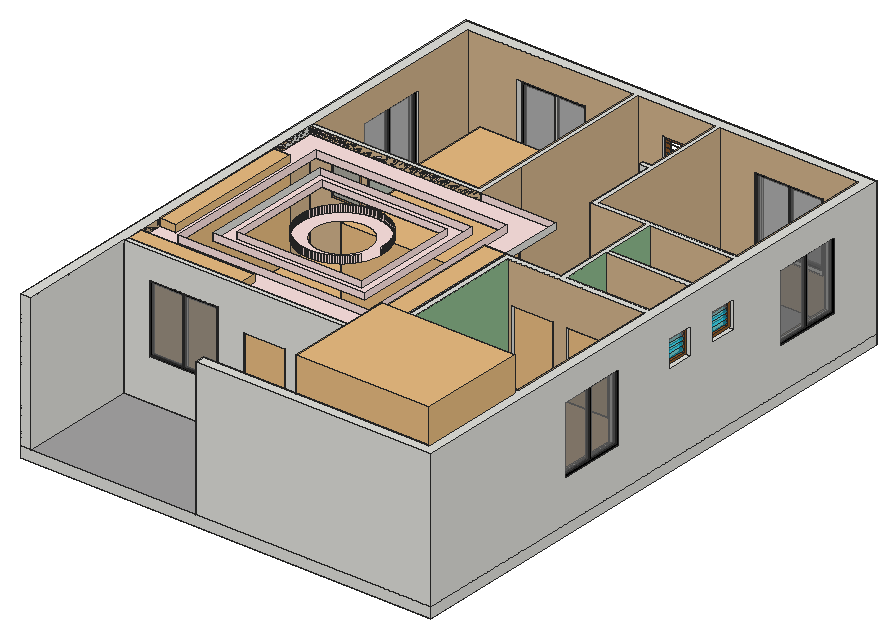
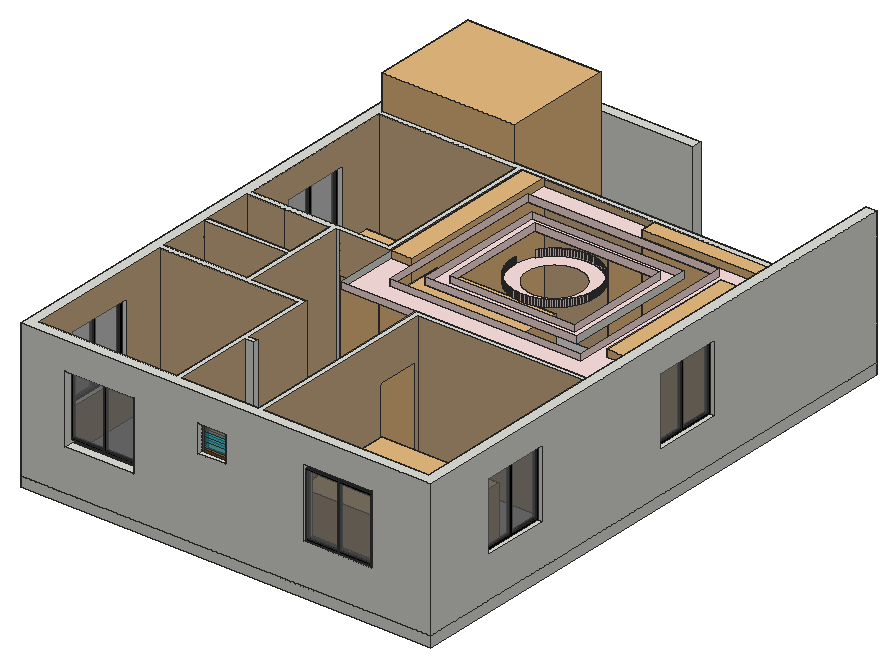
# SketchUp Ruby script. Lengths in inches.
U = 1.inch
M = Sketchup.active_model
def pt(a) = Geom::Point3d.new(a.map { |v| v * U })
def face(e, loops, mat)
  f = e.add_face(loops[0].map { |a| pt(a) })
  loops[1..].each { |l| e.add_face(l.map { |a| pt(a) }).erase! }
  f.material = f.back_material = mat if mat
  f
end
# faces: each face lists its corners as indices into pts; further lists are holes
def faces(e, pts, list, mat = nil) = list.each { |f| face(e, (f[0].is_a?(Array) ? f : [f]).map { |l| l.map { |i| pts[i] } }, mat) }
# xy, xz, yz: faces in a plane at the given z, y or x. An outline is a flat list of corners, or four numbers for a rectangle; further outlines are holes
def ring(l) = l.size == 4 ? [[l[0], l[1]], [l[2], l[1]], [l[2], l[3]], [l[0], l[3]]] : l.each_slice(2).to_a
def flat(e, list, mat, &to3) = list.each { |f| face(e, (f[0].is_a?(Array) ? f : [f]).map { |l| ring(l).map { |u, v| to3.(u, v) } }, mat) }
def xy(e, z, list, mat = nil) = flat(e, list, mat) { |x, y| [x, y, z] }
def xz(e, y, list, mat = nil) = flat(e, list, mat) { |x, z| [x, y, z] }
def yz(e, x, list, mat = nil) = flat(e, list, mat) { |y, z| [x, y, z] }
def lines(e, pts, list) = list.each { |a, b| e.add_line(pt(pts[a]), pt(pts[b])) }
# prism: a flat outline (further loops are holes) pulled along v
def prism(e, loops, v, mat = nil)
  f = face(e, loops, mat); d = Geom::Vector3d.new(v.map { |x| x * U })
  f.pushpull(f.normal.samedirection?(d) ? d.length : -d.length)
end
def box(e, o, s, mat = nil) = prism(e, [[o, [o[0] + s[0], o[1], o[2]], [o[0] + s[0], o[1] + s[1], o[2]], [o[0], o[1] + s[1], o[2]]]], [0, 0, s[2]], mat)
def at(x, y, z, deg = 0) = Geom::Transformation.translation(pt([x, y, z])) * Geom::Transformation.rotation(ORIGIN, Z_AXIS, deg.degrees)
def axes(o, x, y, z) = Geom::Transformation.new([*x, 0, *y, 0, *z, 0, *pt(o).to_a, 1])
def part(name) = M.definitions.add(name)
# library, detail: a bought-in or finely detailed component or shape, given as its bounding box
def library(name, o, s) = part(name).tap { |d| box(d.entities, o, s) }
def detail(e, o, s) = box(e.add_group.entities, o, s)
def put(e, d, t, mat = nil) = e.add_instance(d, t).tap { |i| i.material = mat if mat }
def group(e, t, mat = nil) = e.add_group.tap { |g| g.transformation = t; g.material = mat if mat }.entities
root = M.entities
M.materials.add("F10").color = [176, 183, 172]
M.materials.add("F11").color = [173, 179, 169]
M.materials.add("F20").color = [169, 167, 158]
M.materials.add("Querkus Oak Naturel Adagio _ Architonic1").color = [173, 130, 81]
M.materials.add("[0007_MistyRose]").color = [255, 228, 225]
M.materials.add("[0010_Snow]").color = [255, 250, 250]
M.materials.add("[0035_Tan]").color = [210, 180, 140]
M.materials.add("[0057_DarkKhaki]").color = [189, 183, 107]
M.materials.add("[0072_DarkSeaGreen]").color = [143, 188, 143]
M.materials.add("[Carrera Marble]").color = [207, 207, 207]
M.materials.add("[Color_008]").color = [30, 30, 30]
M.materials.add("[Color_009]").color = [0, 0, 0]
M.materials.add("[Stone Vein Gray]").color = [166, 165, 165]
M.materials.add("[Translucent Glass Gray]").color = [128, 128, 128]
M.materials["[Translucent Glass Gray]"].alpha = 0.5
M.materials.add("[Translucent Glass Tinted]1").color = [7, 201, 240]
M.materials["[Translucent Glass Tinted]1"].alpha = 0.48
M.materials.add("[Translucent_Glass_Gray]").color = [128, 128, 128]
M.materials["[Translucent_Glass_Gray]"].alpha = 0.5
M.materials.add("[Wood Cherry Original]").color = [152, 86, 42]
M.materials.add("[Wood Floor Parquet]").color = [145, 89, 39]
c1 = library("Group\#5",[0,0,0],[116.44,93.99,154.6875])
c2 = library("Senza",[-40.91,-66.2,-0.5],[133.3,90.15,38.26])
c3 = library("Modern+dining",[-0.9,-1.38,-0.1],[126.72,78.33,130.86])
c4 = library("main+door",[0,-0.79,0],[47.24,7.88,82.68])
c5 = library("Bed",[-100.55,9.74,0],[90.43,103.1,58.68])
c6 = library("CS300DRT",[0,0,0],[27.18,17.85,30.31])
c7 = part("ventilator")
g1 = group(c7.entities,at(0,0,0))
xy(g1,0,[[0,0,24,1],[0,1,24,6.83]],"[Wood Floor Parquet]")
xy(g1,1.75,[[2,0,22,6.83]],"[Wood Floor Parquet]")
xy(g1,21.87,[[2,0,22,6.83]],"[Wood Cherry Original]")
xy(g1,23.62,[[0,0,24,1],[0,1,24,6.83]],"[Wood Floor Parquet]")
xz(g1,0,[[[0,0,24,23.62],[2,1.75,22,21.87]]],"[Wood Floor Parquet]")
xz(g1,6.83,[[[0,0,24,23.62],[2,1.75,22,21.87]]],"[Wood Cherry Original]")
yz(g1,0,[[0,0,1,23.62],[1,0,6.83,23.62]],"[Wood Floor Parquet]")
yz(g1,2,[[0,1.75,6.83,1.75,6.83,7.66,0,3.5],[0,3.5,6.83,7.66,6.83,11.8125,0,7.66],[0,7.66,6.83,11.8125,6.83,15.97,0,11.8125],[0,11.8125,6.83,15.97,6.83,20.12,0,15.97],[0,15.97,6.83,20.12,6.83,21.87,0,21.87]],"[Wood Floor Parquet]")
yz(g1,22,[[0,1.75,0,3.5,6.83,7.66,6.83,1.75],[0,3.5,0,7.66,6.83,11.8125,6.83,7.66],[0,7.66,0,11.8125,6.83,15.97,6.83,11.8125],[0,11.8125,0,15.97,6.83,20.12,6.83,15.97],[0,15.97,0,21.87,6.83,21.87,6.83,20.12]],"[Wood Floor Parquet]")
yz(g1,24,[[0,0,1,23.62],[1,0,6.83,23.62]],"[Wood Floor Parquet]")
p = [[2,0,3.5],[2,6.83,7.66],[22,6.83,7.66],[22,0,3.5],[2,6.83,11.8125],[2,0,7.66],
  [22,0,7.66],[22,6.83,11.8125],[2,0,11.8125],[2,6.83,15.97],[22,6.83,15.97],[22,0,11.8125],
  [2,6.83,20.12],[2,0,15.97],[22,0,15.97],[22,6.83,20.12]]
faces(g1,p,[[0,1,2,3],[4,5,6,7],[8,9,10,11]],"[Translucent Glass Tinted]1")
faces(g1,p,[[12,13,14,15]],"[Translucent Glass Gray]")
c8 = part("Group\#2")
xy(c8.entities,0,[[0,0,82.68,1.18]],"[Color_009]")
xy(c8.entities,1.97,[[1.97,0.98,40.35,1.18],[42.32,0.98,80.71,1.18]])
xy(c8.entities,1.97,[[1.97,0,40.35,0.3],[42.32,0,80.71,0.3]],"[Color_009]")
xy(c8.entities,80.71,[[1.97,0,40.35,0.3],[42.32,0,80.71,0.3],[1.97,0.3,40.35,0.98],[42.32,0.3,80.71,0.98],[1.97,0.98,40.35,1.18],
  [42.32,0.98,80.71,1.18]])
xy(c8.entities,82.68,[[0,0,82.68,1.18]],"[Color_008]")
xz(c8.entities,0,[[[0,0,82.68,82.68],[1.97,1.97,40.35,80.71],[42.32,1.97,80.71,80.71]]],"[Color_009]")
xz(c8.entities,0.3,[[1.97,1.97,40.35,80.71],[42.32,1.97,80.71,80.71]],"[Translucent_Glass_Gray]")
xz(c8.entities,0.98,[[1.97,1.97,40.35,80.71],[42.32,1.97,80.71,80.71]],"[Translucent_Glass_Gray]")
xz(c8.entities,1.18,[[[0,0,82.68,82.68],[1.97,1.97,80.71,80.71]],[40.35,1.97,42.32,80.71]],"[Color_009]")
yz(c8.entities,0,[[0,0,1.18,82.68]],"[Color_009]")
yz(c8.entities,1.97,[[0.98,1.97,1.18,80.71]])
yz(c8.entities,1.97,[[0,1.97,0.3,80.71]],"[Color_009]")
yz(c8.entities,40.35,[[0,1.97,0.3,80.71],[0.98,1.97,1.18,80.71]],"[Color_009]")
yz(c8.entities,42.32,[[0,1.97,0.3,80.71],[0.98,1.97,1.18,80.71]])
yz(c8.entities,80.71,[[0,1.97,0.3,80.71],[0.98,1.97,1.18,80.71]],"[Color_009]")
yz(c8.entities,82.68,[[0,0,1.18,82.68]],"[Color_009]")
c9 = library("Group\#28",[0,0,0],[19.5,144,120])
c10 = library("Platform bed",[0,0,0],[83.59,112.46,35.43])
c11 = library("Curtains and rod",[2.63,-1.46,0.02],[153.32,14.02,114.15])
c12 = library("SKT_Nearly Natural 5' Kentia Palm Silk Tree",[-23.18,-17.61,0],[47.48,43.95,59.125])
c13 = library("Round wall hanging",[0,0,0],[26.88,1.18,49.49])
c14 = part("Group\#37")
prism(c14.entities,[[[0,0.6,0],[0,0.6,24.5],[19,0.6,24.5],[19,0.6,0]],[[0.5,0.6,0.5],[18.5,0.6,0.5],[18.5,0.6,24],[0.5,0.6,24]]],[0,-0.6,0])
c15 = part("F9")
g2 = group(c15.entities,at(48,0,0))
xy(g2,0.5,[[0.5,0.3,18.5,0.6]])
xy(g2,24,[[0.5,0.3,18.5,0.6]])
xz(g2,0.3,[[0.5,0.5,18.5,24]],"F11")
xz(g2,0.6,[[0.5,0.5,18.5,24]],"[0010_Snow]")
yz(g2,0.5,[[0.3,0.5,0.6,24]])
yz(g2,18.5,[[0.3,0.5,0.6,24]])
put(g2,c14,axes([19,0,0],[-1,0,0],[0,1,0],[0,0,1]),"Querkus Oak Naturel Adagio _ Architonic1")
g3 = group(c15.entities,at(24,0,0))
xy(g3,0.5,[[0.5,0.3,18.5,0.6]])
xy(g3,24,[[0.5,0.3,18.5,0.6]])
xz(g3,0.3,[[0.5,0.5,18.5,24]],"F10")
xz(g3,0.6,[[0.5,0.5,18.5,24]],"[0010_Snow]")
yz(g3,0.5,[[0.3,0.5,0.6,24]])
yz(g3,18.5,[[0.3,0.5,0.6,24]])
put(g3,c14,axes([19,0,0],[-1,0,0],[0,1,0],[0,0,1]),"Querkus Oak Naturel Adagio _ Architonic1")
g4 = group(c15.entities,at(0,0,0))
xy(g4,0.5,[[0.5,0.3,18.5,0.6]])
xy(g4,24,[[0.5,0.3,18.5,0.6]])
xz(g4,0.3,[[0.5,0.5,18.5,24]],"F20")
xz(g4,0.6,[[0.5,0.5,18.5,24]],"[0010_Snow]")
yz(g4,0.5,[[0.3,0.5,0.6,24]])
yz(g4,18.5,[[0.3,0.5,0.6,24]])
put(g4,c14,axes([19,0,0],[-1,0,0],[0,1,0],[0,0,1]),"Querkus Oak Naturel Adagio _ Architonic1")
xy(root,114,[[[9,107.25,224.75,306.75],[33,131.25,200.75,282.75]],[[50.24,148.49,183.51,265.51],[62.05,160.3,171.7,253.7]],[[116.7,171,115.57,171.02,114.44,171.08,113.3125,171.18,112.19,171.31,111.07,171.47,109.96,171.67,108.85,171.91,107.75,172.17,106.66,172.48,105.58,172.82,104.52,173.1875,103.46,173.59,102.42,174.03,101.39,174.5,100.375,175,99.38,175.54,98.4,176.1,97.4375,176.7,96.5,177.32,95.57,177.98,94.67,178.66,93.79,179.37,92.9375,180.11,92.1,180.875,91.3,181.67,90.51,182.48,89.76,183.32,89.03,184.1875,88.32,185.07,87.65,185.98,87,186.91,86.39,187.86,85.8,188.82,85.24,189.81,84.72,190.8125,84.23,191.83,83.77,192.86,83.34,193.91,82.94,194.97,82.58,196.04,82.26,197.125,81.96,198.22,81.7,199.32,81.48,200.43,81.29,201.54,81.14,202.66,81.02,203.79,80.9375,204.91,80.89,206.04,80.875,207.17,80.9,208.3,80.96,209.43,81.05,210.5625,81.18,211.68,81.35,212.8,81.55,213.92,81.78,215.02,82.05,216.12,82.35,217.21,82.69,218.29,83.0625,219.36,83.47,220.41,83.91,221.46,84.375,222.49,84.88,223.5,85.41,224.5,85.98,225.48,86.57,226.4375,87.2,227.38,87.85,228.3,88.54,229.2,89.25,230.08,89.99,230.9375,90.75,231.77,91.54,232.58,92.36,233.36,93.2,234.12,94.0625,234.85,94.95,235.55,95.86,236.23,96.78,236.87,97.73,237.49,98.7,238.08,99.68,238.63,100.6875,239.15,101.7,239.65,102.74,240.11,103.78,240.54,104.84,240.93,105.92,241.29,107,241.62,108.09,241.91,109.19,242.17,110.3,242.39,111.42,242.58,112.54,242.74,113.66,242.86,114.79,242.9375,115.92,242.99,117.05,243,118.18,242.98,119.31,242.92,120.4375,242.82,121.56,242.69,122.68,242.53,123.79,242.33,124.9,242.09,126,241.83,127.09,241.52,128.17,241.18,129.23,240.8125,130.29,240.41,131.33,239.97,132.36,239.5,133.375,239,134.37,238.46,135.35,237.9,136.3125,237.3,137.25,236.68,138.18,236.02,139.08,235.34,139.96,234.63,140.8125,233.89,141.65,233.125,142.45,232.33,143.24,231.52,143.99,230.68,144.72,229.8125,145.43,228.93,146.1,228.02,146.75,227.09,147.36,226.14,147.95,225.18,148.51,224.19,149.03,223.1875,149.52,222.17,149.98,221.14,150.41,220.09,150.81,219.03,151.17,217.96,151.49,216.875,151.79,215.78,152.05,214.68,152.27,213.57,152.46,212.46,152.61,211.34,152.73,210.21,152.8125,209.09,152.86,207.96,152.875,206.83,152.85,205.7,152.79,204.57,152.7,203.4375,152.57,202.32,152.4,201.2,152.2,200.08,151.97,198.98,151.7,197.88,151.4,196.79,151.06,195.71,150.6875,194.64,150.28,193.59,149.84,192.54,149.375,191.51,148.87,190.5,148.34,189.5,147.77,188.52,147.18,187.5625,146.55,186.62,145.9,185.7,145.21,184.8,144.5,183.92,143.76,183.0625,143,182.23,142.21,181.42,141.39,180.64,140.55,179.88,139.6875,179.15,138.8,178.45,137.89,177.77,136.97,177.13,136.02,176.51,135.05,175.92,134.07,175.37,133.0625,174.85,132.05,174.35,131.01,173.89,129.97,173.46,128.91,173.07,127.83,172.71,126.75,172.38,125.66,172.09,124.56,171.83,123.45,171.61,122.33,171.42,121.21,171.26,120.09,171.14,118.96,171.0625,117.83,171.01],[116.59,183,117.34,183,118.1,183.03,118.85,183.08,119.6,183.15,120.35,183.25,121.09,183.37,121.83,183.52,122.56,183.68,123.29,183.875,124.02,184.09,124.73,184.32,125.44,184.58,126.14,184.86,126.83,185.16,127.51,185.49,128.18,185.83,128.84,186.2,129.49,186.58,130.125,186.99,130.75,187.42,131.36,187.86,131.95,188.33,132.53,188.81,133.09,189.31,133.64,189.83,134.17,190.36,134.6875,190.91,135.18,191.48,135.66,192.0625,136.12,192.66,136.5625,193.27,136.98,193.9,137.39,194.54,137.77,195.1875,138.13,195.85,138.47,196.52,138.79,197.21,139.08,197.9,139.36,198.6,139.61,199.3125,139.84,200.03,140.05,200.75,140.23,201.48,140.39,202.22,140.53,202.96,140.65,203.71,140.74,204.46,140.81,205.21,140.85,205.96,140.875,206.71,140.87,207.47,140.84,208.22,140.79,208.97,140.72,209.72,140.62,210.47,140.5,211.21,140.36,211.95,140.19,212.69,140,213.42,139.79,214.14,139.55,214.86,139.29,215.57,139.01,216.27,138.71,216.96,138.39,217.64,138.04,218.31,137.68,218.97,137.29,219.62,136.89,220.25,136.46,220.875,136.01,221.48,135.55,222.08,135.07,222.65,134.57,223.22,134.05,223.77,133.51,224.3,132.96,224.8125,132.39,225.31,131.8125,225.79,131.21,226.25,130.6,226.6875,129.98,227.11,129.34,227.51,128.6875,227.89,128.03,228.25,127.35,228.59,126.67,228.91,125.98,229.21,125.27,229.48,124.5625,229.73,123.85,229.97,123.12,230.17,122.39,230.36,121.65,230.52,120.91,230.66,120.17,230.77,119.42,230.86,118.67,230.93,117.92,230.98,117.16,231,116.41,231,115.65,230.97,114.9,230.92,114.15,230.85,113.4,230.75,112.66,230.63,111.92,230.48,111.19,230.32,110.46,230.125,109.73,229.91,109.02,229.68,108.31,229.42,107.61,229.14,106.92,228.84,106.24,228.51,105.57,228.17,104.91,227.8,104.26,227.42,103.625,227.01,103,226.58,102.39,226.14,101.8,225.67,101.22,225.19,100.66,224.69,100.11,224.17,99.58,223.64,99.0625,223.09,98.57,222.52,98.09,221.9375,97.63,221.34,97.1875,220.73,96.77,220.1,96.36,219.46,95.98,218.8125,95.62,218.15,95.28,217.48,94.96,216.79,94.67,216.1,94.39,215.4,94.14,214.6875,93.91,213.97,93.7,213.25,93.52,212.52,93.36,211.78,93.22,211.04,93.1,210.29,93.01,209.54,92.94,208.79,92.9,208.04,92.875,207.29,92.88,206.53,92.91,205.78,92.96,205.03,93.03,204.28,93.13,203.53,93.25,202.79,93.39,202.05,93.56,201.31,93.75,200.58,93.96,199.86,94.2,199.14,94.46,198.43,94.74,197.73,95.04,197.04,95.36,196.36,95.71,195.69,96.07,195.03,96.46,194.38,96.86,193.75,97.29,193.125,97.74,192.52,98.2,191.92,98.68,191.35,99.18,190.78,99.7,190.23,100.24,189.7,100.79,189.1875,101.36,188.69,101.9375,188.21,102.54,187.75,103.15,187.3125,103.77,186.89,104.41,186.49,105.0625,186.11,105.72,185.75,106.4,185.41,107.08,185.09,107.77,184.79,108.48,184.52,109.1875,184.27,109.9,184.03,110.63,183.83,111.36,183.64,112.1,183.48,112.84,183.34,113.58,183.23,114.33,183.14,115.08,183.07,115.83,183.02]]],"[0007_MistyRose]")
xz(root,107.25,[[9,114,224.75,120]])
xz(root,131.25,[[33,114,200.75,120]],"[0007_MistyRose]")
xz(root,148.49,[[50.24,114,183.51,120]],"[0007_MistyRose]")
xz(root,160.3,[[62.05,114,171.7,120]],"[0007_MistyRose]")
xz(root,253.7,[[62.05,114,171.7,120]],"[0007_MistyRose]")
xz(root,265.51,[[50.24,114,183.51,120]],"[0007_MistyRose]")
xz(root,282.75,[[33,114,200.75,120]],"[0007_MistyRose]")
xz(root,306.75,[[9,114,224.75,120]],"[0007_MistyRose]")
yz(root,9,[[107.25,114,306.75,120]])
yz(root,33,[[131.25,114,282.75,120]],"[0007_MistyRose]")
yz(root,50.24,[[148.49,114,265.51,120]])
yz(root,62.05,[[160.3,114,253.7,120]],"[0007_MistyRose]")
yz(root,171.7,[[160.3,114,253.7,120]],"[0007_MistyRose]")
yz(root,183.51,[[148.49,114,265.51,120]],"[0007_MistyRose]")
yz(root,200.75,[[131.25,114,282.75,120]],"[0007_MistyRose]")
yz(root,224.75,[[107.25,114,306.75,120]])
p = [[115.57,171.02,120],[114.44,171.08,120],[114.44,171.08,114],[115.57,171.02,114],[116.7,171,120],[116.7,171,114],
  [117.83,171.01,120],[117.83,171.01,114],[118.96,171.0625,120],[118.96,171.0625,114],[113.3125,171.18,120],[113.3125,171.18,114],
  [120.09,171.14,120],[120.09,171.14,114],[121.21,171.26,120],[121.21,171.26,114],[112.19,171.31,120],[112.19,171.31,114],
  [111.07,171.47,120],[111.07,171.47,114],[122.33,171.42,120],[122.33,171.42,114],[123.45,171.61,120],[123.45,171.61,114],
  [109.96,171.67,120],[109.96,171.67,114],[124.56,171.83,120],[124.56,171.83,114],[108.85,171.91,120],[108.85,171.91,114],
  [125.66,172.09,120],[125.66,172.09,114],[107.75,172.17,120],[107.75,172.17,114],[126.75,172.38,120],[126.75,172.38,114],
  [106.66,172.48,120],[106.66,172.48,114],[127.83,172.71,120],[127.83,172.71,114],[105.58,172.82,120],[105.58,172.82,114],
  [128.91,173.07,120],[128.91,173.07,114],[104.52,173.1875,120],[104.52,173.1875,114],[129.97,173.46,120],[129.97,173.46,114],
  [103.46,173.59,120],[103.46,173.59,114],[131.01,173.89,120],[131.01,173.89,114],[102.42,174.03,120],[102.42,174.03,114],
  [132.05,174.35,120],[132.05,174.35,114],[101.39,174.5,120],[101.39,174.5,114],[133.0625,174.85,120],[133.0625,174.85,114],
  [100.375,175,120],[100.375,175,114],[134.07,175.37,120],[134.07,175.37,114],[99.38,175.54,120],[99.38,175.54,114],
  [135.05,175.92,120],[135.05,175.92,114],[98.4,176.1,120],[98.4,176.1,114],[136.02,176.51,120],[136.02,176.51,114],
  [97.4375,176.7,120],[97.4375,176.7,114],[136.97,177.13,120],[136.97,177.13,114],[96.5,177.32,120],[96.5,177.32,114],
  [137.89,177.77,120],[137.89,177.77,114],[95.57,177.98,120],[95.57,177.98,114],[138.8,178.45,120],[138.8,178.45,114],
  [94.67,178.66,120],[94.67,178.66,114],[139.6875,179.15,120],[139.6875,179.15,114],[93.79,179.37,120],[93.79,179.37,114],
  [140.55,179.88,120],[140.55,179.88,114],[92.9375,180.11,120],[92.9375,180.11,114],[141.39,180.64,120],[141.39,180.64,114],
  [92.1,180.875,120],[92.1,180.875,114],[142.21,181.42,120],[142.21,181.42,114],[91.3,181.67,120],[91.3,181.67,114],
  [143,182.23,120],[143,182.23,114],[90.51,182.48,120],[90.51,182.48,114],[143.76,183.0625,120],[143.76,183.0625,114],
  [89.76,183.32,120],[89.76,183.32,114],[144.5,183.92,120],[144.5,183.92,114],[89.03,184.1875,120],[89.03,184.1875,114],
  [145.21,184.8,120],[145.21,184.8,114],[88.32,185.07,120],[88.32,185.07,114],[145.9,185.7,120],[145.9,185.7,114],
  [87.65,185.98,120],[87.65,185.98,114],[146.55,186.62,120],[146.55,186.62,114],[87,186.91,120],[87,186.91,114],
  [147.18,187.5625,120],[147.18,187.5625,114],[86.39,187.86,120],[86.39,187.86,114],[147.77,188.52,120],[147.77,188.52,114],
  [85.8,188.82,120],[85.8,188.82,114],[85.24,189.81,120],[85.24,189.81,114],[84.72,190.8125,120],[84.72,190.8125,114],
  [84.23,191.83,120],[84.23,191.83,114],[83.77,192.86,120],[83.77,192.86,114],[83.34,193.91,120],[83.34,193.91,114],
  [82.94,194.97,120],[82.94,194.97,114],[82.58,196.04,120],[82.58,196.04,114],[82.26,197.125,120],[82.26,197.125,114],
  [81.96,198.22,120],[81.96,198.22,114],[81.7,199.32,120],[81.7,199.32,114],[81.48,200.43,120],[81.48,200.43,114],
  [81.29,201.54,120],[81.29,201.54,114],[81.14,202.66,120],[81.14,202.66,114],[81.02,203.79,120],[81.02,203.79,114],
  [80.9375,204.91,120],[80.9375,204.91,114],[152.85,205.7,120],[152.79,204.57,120],[152.79,204.57,114],[152.85,205.7,114],
  [80.89,206.04,120],[80.89,206.04,114],[152.875,206.83,120],[152.875,206.83,114],[80.875,207.17,120],[80.875,207.17,114],
  [152.86,207.96,120],[152.86,207.96,114],[80.9,208.3,120],[80.9,208.3,114],[152.8125,209.09,120],[152.8125,209.09,114],
  [80.96,209.43,120],[80.96,209.43,114],[152.73,210.21,120],[152.73,210.21,114],[81.05,210.5625,120],[81.05,210.5625,114],
  [152.61,211.34,120],[152.61,211.34,114],[81.18,211.68,120],[81.18,211.68,114],[152.46,212.46,120],[152.46,212.46,114],
  [81.35,212.8,120],[81.35,212.8,114],[152.27,213.57,120],[152.27,213.57,114],[81.55,213.92,120],[81.55,213.92,114],
  [152.05,214.68,120],[152.05,214.68,114],[81.78,215.02,120],[81.78,215.02,114],[151.79,215.78,120],[151.79,215.78,114],
  [82.05,216.12,120],[82.05,216.12,114],[151.49,216.875,120],[151.49,216.875,114],[82.35,217.21,120],[82.35,217.21,114],
  [151.17,217.96,120],[151.17,217.96,114],[82.69,218.29,120],[82.69,218.29,114],[150.81,219.03,120],[150.81,219.03,114],
  [83.0625,219.36,120],[83.0625,219.36,114],[150.41,220.09,120],[150.41,220.09,114],[83.47,220.41,120],[83.47,220.41,114],
  [149.98,221.14,120],[149.98,221.14,114],[83.91,221.46,120],[83.91,221.46,114],[149.52,222.17,120],[149.52,222.17,114],
  [84.375,222.49,120],[84.375,222.49,114],[149.03,223.1875,120],[149.03,223.1875,114],[84.88,223.5,120],[84.88,223.5,114],
  [148.51,224.19,120],[148.51,224.19,114],[85.41,224.5,120],[85.41,224.5,114],[147.95,225.18,120],[147.95,225.18,114],
  [85.98,225.48,120],[85.98,225.48,114],[147.36,226.14,120],[147.36,226.14,114],[86.57,226.4375,120],[86.57,226.4375,114],
  [146.75,227.09,120],[146.75,227.09,114],[87.2,227.38,120],[87.2,227.38,114],[146.1,228.02,120],[146.1,228.02,114],
  [87.85,228.3,120],[87.85,228.3,114],[145.43,228.93,120],[145.43,228.93,114],[88.54,229.2,120],[88.54,229.2,114],
  [144.72,229.8125,120],[144.72,229.8125,114],[89.25,230.08,120],[89.25,230.08,114],[143.99,230.68,120],[143.99,230.68,114],
  [89.99,230.9375,120],[89.99,230.9375,114],[143.24,231.52,120],[143.24,231.52,114],[90.75,231.77,120],[90.75,231.77,114],
  [142.45,232.33,120],[142.45,232.33,114],[91.54,232.58,120],[91.54,232.58,114],[141.65,233.125,120],[141.65,233.125,114],
  [92.36,233.36,120],[92.36,233.36,114],[140.8125,233.89,120],[140.8125,233.89,114],[93.2,234.12,120],[93.2,234.12,114],
  [139.96,234.63,120],[139.96,234.63,114],[94.0625,234.85,120],[94.0625,234.85,114],[139.08,235.34,120],[139.08,235.34,114],
  [94.95,235.55,120],[94.95,235.55,114],[138.18,236.02,120],[138.18,236.02,114],[95.86,236.23,120],[95.86,236.23,114],
  [137.25,236.68,120],[137.25,236.68,114],[96.78,236.87,120],[96.78,236.87,114],[136.3125,237.3,120],[136.3125,237.3,114],
  [97.73,237.49,120],[97.73,237.49,114],[135.35,237.9,120],[135.35,237.9,114],[98.7,238.08,120],[98.7,238.08,114],
  [134.37,238.46,120],[134.37,238.46,114],[99.68,238.63,120],[99.68,238.63,114],[133.375,239,120],[133.375,239,114],
  [100.6875,239.15,120],[100.6875,239.15,114],[132.36,239.5,120],[132.36,239.5,114],[101.7,239.65,120],[101.7,239.65,114],
  [131.33,239.97,120],[131.33,239.97,114],[102.74,240.11,120],[102.74,240.11,114],[130.29,240.41,120],[130.29,240.41,114],
  [103.78,240.54,120],[103.78,240.54,114],[129.23,240.8125,120],[129.23,240.8125,114],[104.84,240.93,120],[104.84,240.93,114],
  [128.17,241.18,120],[128.17,241.18,114],[105.92,241.29,120],[105.92,241.29,114],[127.09,241.52,120],[127.09,241.52,114],
  [107,241.62,120],[107,241.62,114],[126,241.83,120],[126,241.83,114],[108.09,241.91,120],[108.09,241.91,114],
  [124.9,242.09,120],[124.9,242.09,114],[109.19,242.17,120],[109.19,242.17,114],[123.79,242.33,120],[123.79,242.33,114],
  [110.3,242.39,120],[110.3,242.39,114],[122.68,242.53,120],[122.68,242.53,114],[111.42,242.58,120],[111.42,242.58,114],
  [121.56,242.69,120],[121.56,242.69,114],[112.54,242.74,120],[112.54,242.74,114],[113.66,242.86,120],[113.66,242.86,114],
  [120.4375,242.82,120],[120.4375,242.82,114],[119.31,242.92,120],[119.31,242.92,114],[114.79,242.9375,120],[114.79,242.9375,114],
  [115.92,242.99,120],[115.92,242.99,114],[118.18,242.98,120],[118.18,242.98,114],[117.05,243,120],[117.05,243,114],
  [158.25,410.25,0],[158.27,410.25,0],[158.25,405.75,0],[158.27,405.75,0]]
faces(root,p,[[0,1,2,3],[4,0,3,5],[6,4,5,7],[8,6,7,9],[1,10,11,2],[12,8,9,13],[14,12,13,15],[10,16,17,11],
  [16,18,19,17],[20,14,15,21],[22,20,21,23],[18,24,25,19],[26,22,23,27],[24,28,29,25],[30,26,27,31],[28,32,33,29],
  [34,30,31,35],[32,36,37,33],[38,34,35,39],[36,40,41,37],[42,38,39,43],[40,44,45,41],[46,42,43,47],[44,48,49,45],
  [50,46,47,51],[48,52,53,49],[54,50,51,55],[52,56,57,53],[58,54,55,59],[56,60,61,57],[62,58,59,63],[60,64,65,61],
  [66,62,63,67],[64,68,69,65],[70,66,67,71],[68,72,73,69],[74,70,71,75],[72,76,77,73],[78,74,75,79],[76,80,81,77],
  [82,78,79,83],[80,84,85,81],[86,82,83,87],[84,88,89,85],[90,86,87,91],[88,92,93,89],[94,90,91,95],[92,96,97,93],
  [98,94,95,99],[96,100,101,97],[102,98,99,103],[100,104,105,101],[106,102,103,107],[104,108,109,105],[110,106,107,111],[108,112,113,109],
  [114,110,111,115],[112,116,117,113],[118,114,115,119],[116,120,121,117],[122,118,119,123],[120,124,125,121],[126,122,123,127],[124,128,129,125],
  [130,126,127,131],[128,132,133,129],[132,134,135,133],[134,136,137,135],[136,138,139,137],[138,140,141,139],[140,142,143,141],[142,144,145,143],
  [144,146,147,145],[146,148,149,147],[148,150,151,149],[150,152,153,151],[152,154,155,153],[154,156,157,155],[156,158,159,157],[158,160,161,159],
  [160,162,163,161],[164,165,166,167],[162,168,169,163],[170,164,167,171],[168,172,173,169],[174,170,171,175],[172,176,177,173],[178,174,175,179],
  [176,180,181,177],[182,178,179,183],[180,184,185,181],[186,182,183,187],[184,188,189,185],[190,186,187,191],[188,192,193,189],[194,190,191,195],
  [192,196,197,193],[198,194,195,199],[196,200,201,197],[202,198,199,203],[200,204,205,201],[206,202,203,207],[204,208,209,205],[210,206,207,211],
  [208,212,213,209],[214,210,211,215],[212,216,217,213],[218,214,215,219],[216,220,221,217],[222,218,219,223],[220,224,225,221],[226,222,223,227],
  [224,228,229,225],[230,226,227,231],[228,232,233,229],[234,230,231,235],[232,236,237,233],[238,234,235,239],[236,240,241,237],[242,238,239,243],
  [240,244,245,241],[246,242,243,247],[244,248,249,245],[250,246,247,251],[248,252,253,249],[254,250,251,255],[252,256,257,253],[258,254,255,259],
  [256,260,261,257],[262,258,259,263],[260,264,265,261],[266,262,263,267],[264,268,269,265],[270,266,267,271],[268,272,273,269],[274,270,271,275],
  [272,276,277,273],[278,274,275,279],[276,280,281,277],[282,278,279,283],[280,284,285,281],[286,282,283,287],[284,288,289,285],[290,286,287,291],
  [288,292,293,289],[294,290,291,295],[292,296,297,293],[298,294,295,299],[296,300,301,297],[302,298,299,303],[300,304,305,301],[306,302,303,307],
  [304,308,309,305],[310,306,307,311],[308,312,313,309],[314,310,311,315],[312,316,317,313],[318,314,315,319],[316,320,321,317],[322,318,319,323],
  [320,324,325,321],[326,322,323,327],[324,328,329,325],[330,326,327,331],[328,332,333,329],[334,330,331,335],[332,336,337,333],[338,334,335,339],
  [336,340,341,337],[342,338,339,343],[340,344,345,341],[346,342,343,347],[344,348,349,345],[350,346,347,351],[348,352,353,349],[354,350,351,355],
  [352,356,357,353],[356,358,359,357],[360,354,355,361],[362,360,361,363],[358,364,365,359],[364,366,367,365],[368,362,363,369],[366,370,371,367],
  [370,368,369,371]],"[0007_MistyRose]")
lines(root,p,[[372,373],[374,375]])
g5 = group(root,at(0,0,-9))
xy(g5,0,[[0,0,360,489]])
xy(g5,9,[[0,0,360,489]],"[Stone Vein Gray]")
xz(g5,0,[[0,0,360,9]])
xz(g5,489,[[0,0,360,9]])
yz(g5,0,[[0,0,489,9]])
yz(g5,360,[[0,0,489,9]])
put(root,c1,at(235,9,-4.4375))
put(root,c2,at(49.13,193.21,0.31,90))
put(root,c3,axes([96.43,233.41,-0.1],[0.82,0,0],[0,0.82,0],[0,0,0.82]))
put(root,c4,axes([273.75,338.75,0],[0,-0.762,0],[0.42,0,0],[0,0,1.016]))
put(root,c5,at(22.55,363.42,0,-90))
put(root,c4,axes([282.21,248.34,0],[0.762,0,0],[0,0.42,0],[0,0,1.016]))
put(root,c4,axes([233.96,248.34,0],[0.762,0,0],[0,0.42,0],[0,0,1.016]))
put(root,c6,at(350.09,331.57,0,180))
put(root,c6,at(350.09,279.51,0,180))
g6 = group(root,at(0,0,0))
xy(g6,0,[[0,0,9,177],[153.75,0,153.75,9,351,9,351,102.75,149.75,102.75,149.75,107.25,225.75,107.25,225.75,251.25,234.25,251.25,234.25,246.75,230.25,246.75,230.25,107.25,351,107.25,351,207,360,207,360,0],[9,102.75,91.375,107.25],[91.375,102.75,113.75,107.25],[0,177,9,365.625],
  [351,207,351,246.75,318.25,246.75,318.25,251.25,351,251.25,351,261,360,261,360,207],[270.25,246.75,270.25,251.25,273.75,251.25,273.75,302.75,278.25,302.75,278.25,251.25,282.25,251.25,282.25,246.75],[351,261,360,309],[9,306.75,9,311.25,153.75,311.25,153.75,315.25,158.3,315.25,158.3,306.75],[351,309,351,342.75,278.25,342.75,278.25,338.75,273.75,338.75,273.75,342.75,270.25,342.75,270.25,347.25,351,347.25,351,443.625,360,443.625,360,309],
  [225.75,342.75,225.75,406.01,217.75,406.01,217.75,410.25,225.75,410.25,225.75,480,204,480,204,489,320.625,489,320.625,480,230.25,480,230.25,347.25,234.23,347.25,234.23,342.75],[153.75,351.25,153.75,480,111.375,480,111.375,489,204,489,204,480,158.21,480,158.21,351.25],[0,365.625,0,489,111.375,489,111.375,480,9,480,9,365.625],[351,443.625,351,480,320.625,480,320.625,489,360,489,360,443.625]])
xy(g6,36,[[31.375,102.75,91.375,107.25],[351,147,360,207],[0,177,9,237],[0,365.625,9,425.625],[351,383.625,360,443.625],
  [51.375,480,111.375,489],[260.625,480,320.625,489]])
xy(g6,72,[[351,261,360,285],[351,309,360,333],[180,480,204,489]])
xy(g6,84,[[113.75,102.75,149.75,107.25],[234.25,246.75,270.25,251.25],[282.25,246.75,318.25,251.25],[273.75,302.75,278.25,338.75],[153.75,315.25,158.21,351.25],
  [158.21,315.25,158.3,351.25],[234.23,342.75,270.25,347.25]])
xy(g6,96,[[351,147,360,207],[0,177,9,237],[351,261,360,285],[351,309,360,333],[0,365.625,9,425.625],
  [351,383.625,360,443.625],[51.375,480,111.375,489],[180,480,204,489],[260.625,480,320.625,489]])
xy(g6,96.36,[[31.375,102.75,91.375,107.25]])
xy(g6,120,[[[0,0,9,0,9,480,153.75,480,153.75,311.25,9,311.25,9,306.75,158.3,306.75,158.3,351.25,158.21,351.25,158.21,480,225.75,480,225.75,410.25,217.75,410.25,217.75,406.01,225.75,406.01,225.75,342.75,273.75,342.75,273.75,251.25,225.75,251.25,225.75,107.25,9,107.25,9,102.75,351,102.75,351,9,153.75,9,153.75,0,360,0,360,489,0,489],[230.25,107.25,351,246.75],[230.25,347.25,351,480],[278.25,251.25,351,342.75]],[278.25,294.75,351,299.25]])
xz(g6,0,[[0,0,9,120],[153.75,0,360,120]])
xz(g6,9,[[153.75,0,351,120]])
xz(g6,102.75,[[[9,0,113.75,0,113.75,84,149.75,84,149.75,0,351,0,351,120,9,120],[31.375,36,91.375,96.36]]])
xz(g6,107.25,[[91.375,0,91.375,120,225.75,120,225.75,0,149.75,0,149.75,84,113.75,84,113.75,0],[230.25,0,351,120]],"[0035_Tan]")
xz(g6,107.25,[[9,0,9,120,91.375,120,91.375,96.36,31.375,96.36,31.375,36,91.375,36,91.375,0]],"[0057_DarkKhaki]")
xz(g6,147,[[351,36,360,96]])
xz(g6,177,[[0,36,9,96]])
xz(g6,207,[[351,36,360,96]])
xz(g6,237,[[0,36,9,96]])
xz(g6,246.75,[[230.25,0,234.25,0,234.25,84,270.25,84,270.25,0,282.25,0,282.25,84,318.25,84,318.25,0,351,0,351,120,230.25,120]],"[0035_Tan]")
xz(g6,251.25,[[270.25,0,273.75,120]])
xz(g6,251.25,[[225.75,0,225.75,120,270.25,120,270.25,84,234.25,84,234.25,0],[278.25,0,278.25,120,318.25,120,318.25,84,282.25,84,282.25,0],[318.25,0,351,120]],"[0035_Tan]")
xz(g6,261,[[351,72,360,96]])
xz(g6,285,[[351,72,360,96]])
xz(g6,294.75,[[278.25,0,351,120]],"[0035_Tan]")
xz(g6,299.25,[[278.25,0,351,120]],"[0035_Tan]")
xz(g6,302.75,[[273.75,0,278.25,84]])
xz(g6,306.75,[[9,0,158.3,120]],"[0035_Tan]")
xz(g6,309,[[351,72,360,96]])
xz(g6,311.25,[[9,0,153.75,120]],"[0035_Tan]")
xz(g6,315.25,[[153.75,0,158.3,84]])
xz(g6,333,[[351,72,360,96]])
xz(g6,338.75,[[273.75,0,278.25,84]])
xz(g6,342.75,[[225.75,0,234.23,0,234.23,84,270.25,84,270.25,0,273.75,0,273.75,120,225.75,120],[278.25,0,351,120]],"[0035_Tan]")
xz(g6,347.25,[[230.25,0,230.25,120,351,120,351,0,270.25,0,270.25,84,234.23,84,234.23,0]],"[0035_Tan]")
xz(g6,351.25,[[153.75,0,158.21,84],[158.21,84,158.3,120]])
xz(g6,365.625,[[0,36,9,96]])
xz(g6,383.625,[[351,36,360,96]])
xz(g6,406.01,[[217.75,0,225.75,120]])
xz(g6,410.25,[[217.75,0,225.75,120]])
xz(g6,425.625,[[0,36,9,96]])
xz(g6,443.625,[[351,36,360,96]])
xz(g6,480,[[[9,0,153.75,120],[51.375,36,111.375,96]],[[158.21,0,225.75,120],[180,72,204,96]],[[230.25,0,351,120],[260.625,36,320.625,96]]],"[0035_Tan]")
xz(g6,489,[[[0,0,360,120],[260.625,36,320.625,96],[51.375,36,111.375,96],[180,72,204,96]]])
yz(g6,0,[[[0,0,489,120],[365.625,36,425.625,96],[177,36,237,96]]])
yz(g6,9,[[0,0,102.75,120],[102.75,0,107.25,120],[306.75,0,311.25,120]])
yz(g6,9,[[[107.25,0,306.75,120],[177,36,237,96]],[[311.25,0,480,120],[365.625,36,425.625,96]]],"[0035_Tan]")
yz(g6,31.375,[[102.75,36,107.25,96.36]])
yz(g6,51.375,[[480,36,489,96]])
yz(g6,91.375,[[102.75,36,107.25,96.36]])
yz(g6,111.375,[[480,36,489,96]])
yz(g6,113.75,[[102.75,0,107.25,84]])
yz(g6,149.75,[[102.75,0,107.25,84]])
yz(g6,153.75,[[0,0,9,120]])
yz(g6,153.75,[[311.25,0,311.25,120,480,120,480,0,351.25,0,351.25,84,315.25,84,315.25,0]],"[0035_Tan]")
yz(g6,158.21,[[351.25,0,480,120]],"[0035_Tan]")
yz(g6,158.3,[[306.75,0,315.25,0,315.25,84,351.25,84,351.25,120,306.75,120]],"[0035_Tan]")
yz(g6,180,[[480,72,489,96]])
yz(g6,204,[[480,72,489,96]])
yz(g6,217.75,[[406.01,0,410.25,120]])
yz(g6,225.75,[[342.75,0,406.01,120],[410.25,0,480,120]],"[0035_Tan]")
yz(g6,225.75,[[107.25,0,251.25,120]],"[Carrera Marble]")
yz(g6,230.25,[[347.25,0,480,120]],"[0035_Tan]")
yz(g6,230.25,[[107.25,0,246.75,120]],"[0072_DarkSeaGreen]")
yz(g6,234.23,[[342.75,0,347.25,84]])
yz(g6,234.25,[[246.75,0,251.25,84]])
yz(g6,260.625,[[480,36,489,96]])
yz(g6,270.25,[[246.75,0,251.25,84],[342.75,0,347.25,84]])
yz(g6,273.75,[[251.25,0,251.25,120,342.75,120,342.75,0,338.75,0,338.75,84,302.75,84,302.75,0]],"[0035_Tan]")
yz(g6,278.25,[[251.25,0,294.75,120],[299.25,0,302.75,0,302.75,84,338.75,84,338.75,0,342.75,0,342.75,120,299.25,120]],"[0072_DarkSeaGreen]")
yz(g6,282.25,[[246.75,0,251.25,84]])
yz(g6,318.25,[[246.75,0,251.25,84]])
yz(g6,320.625,[[480,36,489,96]])
yz(g6,351,[[9,0,102.75,120],[294.75,0,299.25,120]])
yz(g6,351,[[[107.25,0,246.75,120],[147,36,207,96]],[[251.25,0,294.75,120],[261,72,285,96]],[[299.25,0,342.75,120],[309,72,333,96]],[[347.25,0,480,120],[383.625,36,443.625,96]]],"[0035_Tan]")
yz(g6,360,[[[0,0,489,120],[383.625,36,443.625,96],[147,36,207,96],[261,72,285,96],[309,72,333,96]]])
put(g6,c7,axes([356.45,261,72.58],[0,1,0],[-0.5,0,0],[0,0,1]))
put(g6,c4,axes([273.02,338.75,0],[0,-0.762,0],[0.42,0,0],[0,0,1.016]))
put(g6,c4,axes([153.875,351.21,0],[0,-0.762,0],[0.42,0,0],[0,0,1.016]))
put(g6,c4,axes([113.75,104.34,0],[0.762,0,0],[0,0.42,0],[0,0,1.016]))
put(g6,c7,axes([356.45,309,72.58],[0,1,0],[-0.5,0,0],[0,0,1]))
put(g6,c7,axes([204,484.5,72],[-1,0,0],[0,-0.5,0],[0,0,1]))
put(g6,c4,axes([234.14,344.17,0],[0.762,0,0],[0,0.42,0],[0,0,1.016]))
put(g6,c8,axes([52.26,484.5,36],[0.715,0,0],[0,2.65,0],[0,0,0.6844]))
put(g6,c8,axes([4.5,237,36],[0,-0.72571,0],[2.65,0,0],[0,0,0.72546]))
put(g6,c8,axes([31.08,102.75,36],[0.7293,0,0],[0,2.65,0],[0,0,0.73231]))
put(g6,c8,axes([355.5,207,36],[0,-0.72571,0],[2.65,0,0],[0,0,0.72571]))
put(g6,c8,axes([355.5,443.625,36],[0,-0.72571,0],[2.65,0,0],[0,0,0.72571]))
put(g6,c8,axes([4.5,424.74,36],[0,-0.715,0],[2.65,0,0],[0,0,0.72571]))
put(g6,c8,axes([261.51,480,39.6],[0.715,0,0],[0,2.65,0],[0,0,0.6844]))
put(root,c9,at(206.25,107.25,0))
put(root,c10,at(268.76,120.84,0))
put(root,c11,axes([10.46,268.91,5.83],[0,-0.8151,0],[1,0,0],[0,0,1]))
put(root,c11,axes([7.29,108.71,5.83],[0.65,0,0],[0,1,0],[0,0,1]))
put(root,c12,axes([213.79,214.89,23.75],[0.65,0,0],[0,0.65,0],[0,0,0.65]))
put(root,c13,axes([124.94,304.29,55.15],[0.71,0,0],[0,2.5702,0],[0,0,0.71]))
put(root,c15,axes([28.35,306.15,71.47],[1.3144,0,0],[0,1.24,0],[0,0,1.3268]))
